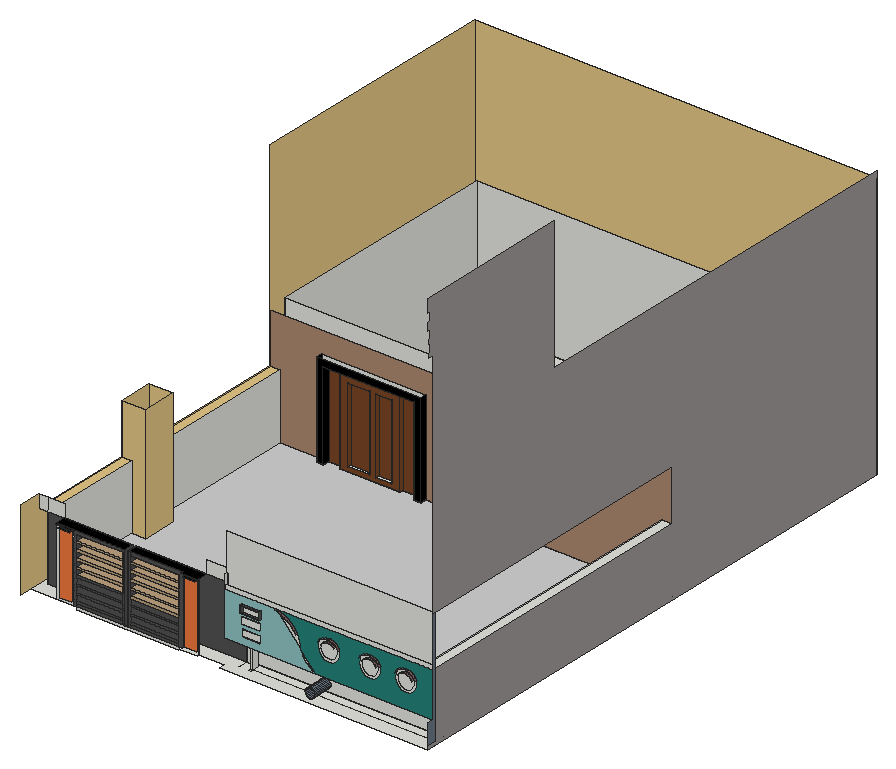
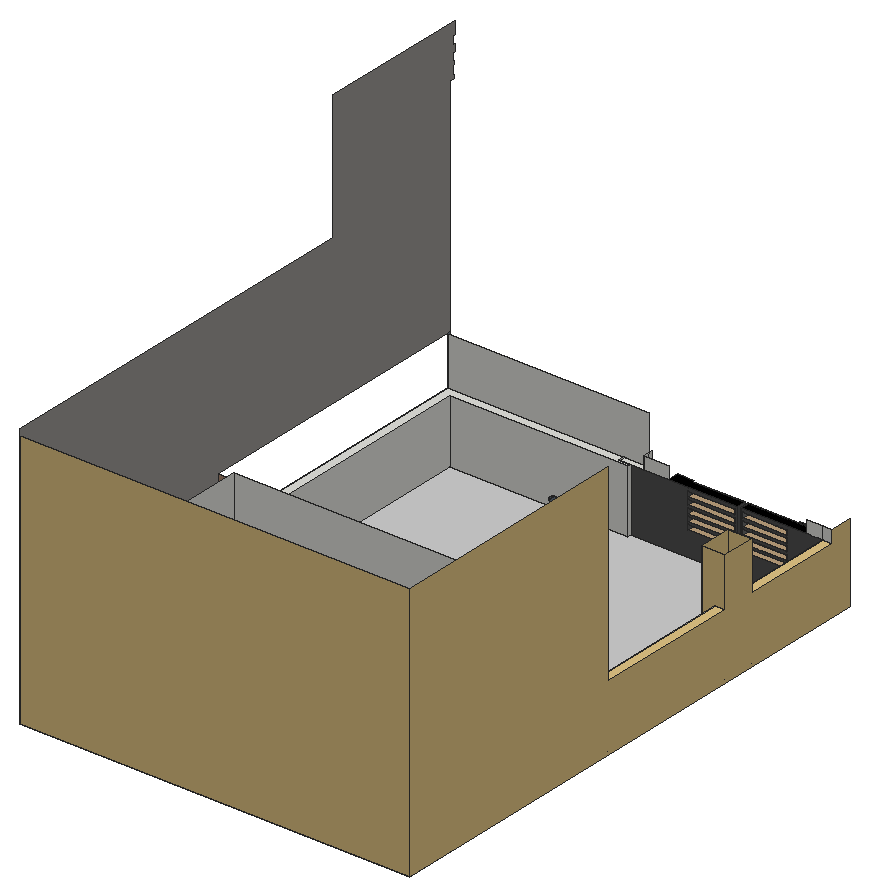
# SketchUp Ruby script. Lengths in inches.
U = 1.inch
M = Sketchup.active_model
def pt(a) = Geom::Point3d.new(a.map { |v| v * U })
def face(e, loops, mat)
  f = e.add_face(loops[0].map { |a| pt(a) })
  loops[1..].each { |l| e.add_face(l.map { |a| pt(a) }).erase! }
  f.material = f.back_material = mat if mat
  f
end
# faces: each face lists its corners as indices into pts; further lists are holes
def faces(e, pts, list, mat = nil) = list.each { |f| face(e, (f[0].is_a?(Array) ? f : [f]).map { |l| l.map { |i| pts[i] } }, mat) }
# xy, xz, yz: faces in a plane at the given z, y or x. An outline is a flat list of corners, or four numbers for a rectangle; further outlines are holes
def ring(l) = l.size == 4 ? [[l[0], l[1]], [l[2], l[1]], [l[2], l[3]], [l[0], l[3]]] : l.each_slice(2).to_a
def flat(e, list, mat, &to3) = list.each { |f| face(e, (f[0].is_a?(Array) ? f : [f]).map { |l| ring(l).map { |u, v| to3.(u, v) } }, mat) }
def xy(e, z, list, mat = nil) = flat(e, list, mat) { |x, y| [x, y, z] }
def xz(e, y, list, mat = nil) = flat(e, list, mat) { |x, z| [x, y, z] }
def yz(e, x, list, mat = nil) = flat(e, list, mat) { |y, z| [x, y, z] }
def lines(e, pts, list) = list.each { |a, b| e.add_line(pt(pts[a]), pt(pts[b])) }
# prism: a flat outline (further loops are holes) pulled along v
def prism(e, loops, v, mat = nil)
  f = face(e, loops, mat); d = Geom::Vector3d.new(v.map { |x| x * U })
  f.pushpull(f.normal.samedirection?(d) ? d.length : -d.length)
end
def box(e, o, s, mat = nil) = prism(e, [[o, [o[0] + s[0], o[1], o[2]], [o[0] + s[0], o[1] + s[1], o[2]], [o[0], o[1] + s[1], o[2]]]], [0, 0, s[2]], mat)
def at(x, y, z, deg = 0) = Geom::Transformation.translation(pt([x, y, z])) * Geom::Transformation.rotation(ORIGIN, Z_AXIS, deg.degrees)
def axes(o, x, y, z) = Geom::Transformation.new([*x, 0, *y, 0, *z, 0, *pt(o).to_a, 1])
def part(name) = M.definitions.add(name)
# library, detail: a bought-in or finely detailed component or shape, given as its bounding box
def library(name, o, s) = part(name).tap { |d| box(d.entities, o, s) }
def detail(e, o, s) = box(e.add_group.entities, o, s)
def put(e, d, t, mat = nil) = e.add_instance(d, t).tap { |i| i.material = mat if mat }
def group(e, t, mat = nil) = e.add_group.tap { |g| g.transformation = t; g.material = mat if mat }.entities
root = M.entities
M.materials.add("[0035_Tan]").color = [186, 159, 124]
M.materials.add("[0035_Tan]1").color = [210, 180, 140]
M.materials.add("[0085_Turquoise]").color = [37, 130, 120]
M.materials.add("[0089_PaleTurquoise]").color = [142, 193, 193]
M.materials.add("[0111_SlateGray]").color = [103, 117, 132]
M.materials.add("[0119_RosyBrown]1").color = [124, 95, 95]
M.materials.add("[0134_DimGray]").color = [105, 105, 105]
M.materials.add("[0135_DarkGray]").color = [81, 81, 81]
M.materials.add("[0137_Black]").color = [0, 0, 0]
M.materials.add("[Carrera Marble]").color = [207, 207, 207]
M.materials.add("[Cast-in-place Concrete]").color = [239, 119, 61]
M.materials.add("[Concrete Aggregate Smoke]").color = [154, 150, 148]
M.materials.add("[Stone Brushed Khaki]").color = [226, 197, 133]
M.materials.add("[Tile Veriegated Stone]").color = [171, 137, 112]
M.materials.add("[Wood Veneer 01]").color = [120, 70, 37]
xy(root,0,[[186.0625,645.11,186.0625,651.11,162.54,651.11,162.54,649.11,146.95,649.11,146.95,651.11,96.94,651.11,96.94,660.11,93.94,660.11,93.94,651.11,7,651.11,7,927.36,54.84,927.36,54.84,921.36,60.84,921.36,60.84,927.36,73.93,927.36,73.93,924.36,129.08,924.36,129.08,927.36,144.84,927.36,144.84,921.36,150.84,921.36,150.84,927.36,377.9375,927.36,377.9375,645.11],[93.94,651.11,96.94,660.11],[54.84,921.36,60.84,927.36],[144.84,921.36,150.84,927.36],[73.93,924.36,129.08,927.36],
  [[7,927.36,377.9375,1163.11],[16,933.36,358,1154.11]],[16,933.36,358,1154.11]])
xy(root,3,[[16,660.11,198.9375,660.11,198.9375,663.11,368.9375,663.11,368.9375,927.36,150.84,927.36,150.84,921.36,144.84,921.36,144.84,927.36,129.08,927.36,129.08,924.36,73.93,924.36,73.93,927.36,60.84,927.36,60.84,921.36,54.84,921.36,54.84,927.36,16,927.36,16,787.78,29,787.78,29,756.09,16,756.09]],"[Carrera Marble]")
xy(root,7.2,[[81.13,924.36,101.5,927.36],[107.04,924.36,121.875,927.36]])
xy(root,26.4,[[49.92,651.11,91.67,660.11],[99.37,651.11,143.95,660.11]],"[0035_Tan]")
xy(root,31.5,[[49.92,651.11,91.67,660.11]],"[0035_Tan]")
xy(root,31.5,[[99.37,651.11,143.95,660.11]],"[0035_Tan]1")
xy(root,33.52,[[49.92,651.11,91.67,660.11],[99.37,651.11,143.95,660.11]],"[0035_Tan]")
xy(root,38.625,[[49.92,651.11,91.67,660.11]],"[0035_Tan]")
xy(root,38.625,[[99.37,651.11,143.95,660.11]],"[0035_Tan]1")
xy(root,40.65,[[49.92,651.11,91.67,660.11],[99.37,651.11,143.95,660.11]],"[0035_Tan]")
xy(root,45.75,[[49.92,651.11,91.67,660.11]],"[0035_Tan]")
xy(root,45.75,[[99.37,651.11,143.95,660.11]],"[0035_Tan]1")
xy(root,47.77,[[49.92,651.11,91.67,660.11],[99.37,651.11,143.95,660.11]],"[0035_Tan]")
xy(root,49.0625,[[201.56,649.11,219.5,651.11]],"[0135_DarkGray]")
xy(root,49.82,[[202.32,649.11,218.74,651.11]],"[0135_DarkGray]")
xy(root,52.875,[[49.92,651.11,91.67,660.11],[99.37,651.11,143.95,660.11]],"[0035_Tan]")
xy(root,54.9,[[49.92,651.11,91.67,660.11],[99.37,651.11,143.95,660.11]],"[0035_Tan]")
xy(root,55.55,[[202.32,649.11,218.74,651.11]],"[0135_DarkGray]")
xy(root,56.3125,[[201.56,649.11,219.5,651.11]],"[0135_DarkGray]")
xy(root,60,[[49.92,651.11,91.67,660.11],[99.37,651.11,143.95,660.11]],"[0135_DarkGray]")
xy(root,60.7,[[33.63,649.11,44.62,651.11]],"[0137_Black]")
xy(root,60.93,[[149.02,649.11,160.48,651.11]],"[0137_Black]")
xy(root,63,[[186.0625,651.11,186.19,654.11],[186.19,651.11,209.625,654.11],[186.19,654.11,209.625,660.11],[209.625,654.11,377.9375,654.11,377.9375,927.36,368.9375,927.36,368.9375,663.11,198.9375,663.11,198.9375,660.11,209.625,660.11]])
xy(root,63,[[31.33,649.11,46.92,651.11],[146.95,649.11,162.54,649.11,162.54,651.11,162.58,651.11,162.58,660.11,96.94,660.11,96.94,651.11,146.95,651.11],[31.33,651.11,93.94,660.11]],"[0137_Black]")
xy(root,63,[[7,660.11,16,756.09],[7,787.78,16,927.36]],"[Stone Brushed Khaki]")
xz(root,651.11,[[49.92,-2.1,143.95,0],[[31.33,0,46.92,63],[33.63,2.3,44.62,60.7]],[162.54,0,162.58,63],[202.42,29.54,218.64,35.08],[282.78,38.68,284.61,39.03,286.28,39.84,287.68,41.0625,288.72,42.6,289.33,44.36,289.46,46.22,289.11,48.04,288.29,49.72,287.07,51.12,285.53,52.16,283.77,52.77,281.92,52.9,280.09,52.55,278.42,51.73,277.02,50.51,275.98,48.97,275.37,47.21,275.24,45.36,275.59,43.53,276.41,41.86,277.625,40.46,279.17,39.41,280.92,38.81],
  [320.72,38.68,322.54,39.03,324.22,39.84,325.62,41.0625,326.66,42.6,327.27,44.36,327.4,46.22,327.05,48.04,326.23,49.72,325.01,51.12,323.47,52.16,321.71,52.77,319.86,52.9,318.03,52.55,316.36,51.73,314.95,50.51,313.91,48.97,313.31,47.21,313.18,45.36,313.53,43.53,314.34,41.86,315.5625,40.46,317.1,39.41,318.86,38.81],[353.97,38.68,355.79,39.03,357.47,39.84,358.87,41.0625,359.91,42.6,360.52,44.36,360.65,46.22,360.3,48.04,359.48,49.72,358.26,51.12,356.72,52.16,354.96,52.77,353.11,52.9,351.28,52.55,349.61,51.73,348.2,50.51,347.16,48.97,346.56,47.21,346.43,45.36,346.78,43.53,347.59,41.86,348.8125,40.46,350.35,39.41,352.11,38.81],[202.31,39.62,218.75,45.375],[202.32,49.82,218.74,55.55],[186.0625,63,377.9375,67.2]])
xz(root,651.11,[[99.37,24.375,143.95,26.4],[49.92,31.5,91.67,33.52],[99.37,31.5,143.95,33.52],[49.92,38.625,91.67,40.65],[99.37,38.625,143.95,40.65],
  [49.92,45.75,91.67,47.77],[99.37,45.75,143.95,47.77],[49.92,52.875,91.67,54.9],[99.37,52.875,143.95,54.9]],"[0035_Tan]")
xz(root,651.11,[[[270.01,22.19,377.9375,22.19,377.9375,63,233.66,63,236.68,62.29,239.6,61.26,242.39,59.9,245.01,58.24,247.43,56.31,249.62,54.11,251.55,51.68,253.19,49.06,254.54,46.26,255.56,43.34,256.26,40.32,256.61,37.24,256.72,37.33,270.11,22.28],[282.96,35.68,280.32,35.87,277.83,36.73,275.64,38.21,273.9,40.21,272.75,42.58,272.24,45.18,272.43,47.8125,273.29,50.3125,274.77,52.5,276.77,54.24,279.14,55.39,281.74,55.9,284.375,55.71,286.875,54.85,289.0625,53.37,290.8,51.37,291.95,48.99,292.46,46.4,292.27,43.76,291.41,41.26,289.93,39.07,287.93,37.34,285.56,36.18],[320.9,35.68,318.26,35.87,315.76,36.73,313.57,38.21,311.84,40.21,310.68,42.58,310.18,45.18,310.37,47.8125,311.23,50.3125,312.71,52.5,314.7,54.24,317.08,55.39,319.68,55.9,322.3125,55.71,324.8125,54.85,327,53.37,328.73,51.37,329.89,48.99,330.39,46.4,330.21,43.76,329.35,41.26,327.87,39.07,325.87,37.34,323.49,36.18],[354.15,35.68,351.51,35.87,349.01,36.73,346.82,38.21,345.09,40.21,343.93,42.58,343.43,45.18,343.62,47.8125,344.48,50.3125,345.96,52.5,347.95,54.24,350.33,55.39,352.93,55.9,355.5625,55.71,358.0625,54.85,360.25,53.37,361.98,51.37,363.14,48.99,363.64,46.4,363.46,43.76,362.6,41.26,361.12,39.07,359.12,37.34,356.74,36.18]]],"[0085_Turquoise]")
xz(root,651.11,[[[186.0625,22.19,270.01,22.19,268.33,22.75,266.71,23.47,265.17,24.34,263.71,25.35,262.36,26.49,261.12,27.76,260,29.14,259.02,30.61,258.1875,32.18,257.5,33.8125,256.97,35.5,256.61,37.24,233.66,63,186.0625,63],[201.56,49.0625,219.5,56.3125],[201.56,38.875,219.5,46.125],[201.56,28.6875,219.5,35.9375]]],"[0089_PaleTurquoise]")
xz(root,651.11,[[46.92,0,49.92,0,49.92,60,91.67,60,91.67,0,93.94,0,93.94,63,46.92,63],[49.92,0,91.67,3],[96.94,0,99.37,63],[143.95,0,146.95,0,146.95,63,99.37,63,99.37,60,143.95,60],[99.37,0,143.95,3],
  [49.92,3,91.67,5.02],[99.37,3,143.95,5.02],[49.92,5.02,91.67,10.125],[99.37,5.02,143.95,10.125],[49.92,10.125,91.67,12.15],
  [99.37,10.125,143.95,12.15],[49.92,12.15,91.67,17.25],[99.37,12.15,143.95,17.25],[49.92,17.25,91.67,19.27],[99.37,17.25,143.95,19.27],
  [49.92,19.27,91.67,24.375],[99.37,19.27,143.95,24.375],[49.92,24.375,91.67,26.4]],"[0135_DarkGray]")
xz(root,651.11,[[149.02,2.07,160.48,60.93],[33.63,2.3,44.62,60.7]],"[Cast-in-place Concrete]")
xz(root,654.11,[[207.9375,3,209.625,63],[186.0625,63,186.19,75],[186.19,63,186.19,75,186.0625,75,186.0625,109.5,377.9375,109.5,377.9375,63]])
xz(root,660.11,[[93.94,0,96.94,3],[198.9375,3,209.625,63],[7,63,16,75],[16,63,31.33,75],[162.58,63,186.19,75]])
xz(root,660.11,[[[16,3,93.94,63],[49.92,54.9,91.67,60],[49.92,47.77,91.67,52.875],[49.92,40.65,91.67,45.75],[49.92,33.52,91.67,38.625],[49.92,26.4,91.67,31.5]],[[96.94,3,198.9375,63],[99.37,26.4,143.95,31.5],[99.37,54.9,143.95,60],[99.37,47.77,143.95,52.875],[99.37,40.65,143.95,45.75],[99.37,33.52,143.95,38.625]]],"[0135_DarkGray]")
xz(root,663.11,[[[198.9375,3,368.9375,63],[269.68,4.18,270.85,4.33,271.93,4.78,272.87,5.5,273.58,6.43,274.03,7.52,274.18,8.68,274.03,9.85,273.58,10.93,272.87,11.86,271.93,12.58,270.85,13.03,269.68,13.18,268.52,13.03,267.43,12.58,266.5,11.86,265.79,10.93,265.34,9.85,265.18,8.68,265.34,7.52,265.79,6.43,266.5,5.5,267.43,4.78,268.52,4.33]]])
xz(root,756.09,[[16,3,29,3,29,109.5,7,109.5,7,63,16,63]],"[Stone Brushed Khaki]")
xz(root,787.78,[[16,3,16,63,7,63,7,109.5,29,109.5,29,3]],"[Stone Brushed Khaki]")
xz(root,921.36,[[54.84,0,60.84,3],[144.84,0,150.84,3]])
xz(root,921.36,[[54.84,3,60.84,3,60.84,84,144.84,84,144.84,3,150.84,3,150.84,90,54.84,90]],"[0137_Black]")
xz(root,924.36,[[73.93,0,129.08,3]])
xz(root,924.36,[[[73.93,3,129.08,84],[81.13,7.2,101.5,76.8],[107.04,7.2,121.875,76.8]]],"[Wood Veneer 01]")
xz(root,927.36,[[60.84,0,73.93,3],[129.08,0,144.84,3],[150.84,0,367,3]])
xz(root,927.36,[[16,3,54.84,3,54.84,90,150.84,90,150.84,3,368.9375,3,368.9375,63,377.9375,63,377.9375,109.5,7,109.5,7,63,16,63]],"[Tile Veriegated Stone]")
xz(root,927.36,[[60.84,3,73.93,84],[129.08,3,144.84,84],[81.13,7.2,101.5,76.8],[107.04,7.2,121.875,76.8]],"[Wood Veneer 01]")
xz(root,933.36,[[16,0,358,120]])
xz(root,1154.11,[[16,0,358,120]])
xz(root,1163.11,[[7,0,377.9375,245.51]],"[Stone Brushed Khaki]")
yz(root,7,[[639.11,0,639.11,75,660.11,75,660.11,63,756.09,63,756.09,109.5,787.78,109.5,787.78,63,927.36,63,927.36,245.51,1163.11,245.51,1163.11,0]],"[Stone Brushed Khaki]")
yz(root,16,[[933.36,0,1154.11,120],[660.11,3,756.09,63],[787.78,3,927.36,63]])
yz(root,29,[[756.09,3,787.78,109.5]],"[Stone Brushed Khaki]")
yz(root,49.92,[[651.11,26.4,660.11,31.5],[651.11,33.52,660.11,38.625],[651.11,40.65,660.11,45.75],[651.11,47.77,660.11,52.875],[651.11,54.9,660.11,60]],"[0135_DarkGray]")
yz(root,54.84,[[921.36,0,927.36,3]])
yz(root,54.84,[[921.36,3,927.36,90]],"[0137_Black]")
yz(root,60.84,[[921.36,0,927.36,3]])
yz(root,60.84,[[921.36,3,927.36,84]],"[0137_Black]")
yz(root,73.93,[[924.36,0,927.36,3]])
yz(root,73.93,[[924.36,3,927.36,84]],"[Wood Veneer 01]")
yz(root,81.13,[[924.36,7.2,927.36,76.8]],"[Wood Veneer 01]")
yz(root,91.67,[[651.11,26.4,660.11,31.5],[651.11,33.52,660.11,38.625],[651.11,40.65,660.11,45.75],[651.11,47.77,660.11,52.875],[651.11,54.9,660.11,60]],"[0134_DimGray]")
yz(root,93.94,[[651.11,0,660.11,63]],"[0135_DarkGray]")
yz(root,96.94,[[651.11,0,660.11,63]],"[0135_DarkGray]")
yz(root,99.37,[[651.11,26.4,660.11,31.5],[651.11,33.52,660.11,38.625],[651.11,40.65,660.11,45.75],[651.11,47.77,660.11,52.875],[651.11,54.9,660.11,60]],"[0135_DarkGray]")
yz(root,101.5,[[924.36,7.2,927.36,76.8]],"[Wood Veneer 01]")
yz(root,107.04,[[924.36,7.2,927.36,76.8]],"[Wood Veneer 01]")
yz(root,121.875,[[924.36,7.2,927.36,76.8]],"[Wood Veneer 01]")
yz(root,129.08,[[924.36,0,927.36,3]])
yz(root,129.08,[[924.36,3,927.36,84]],"[Wood Veneer 01]")
yz(root,143.95,[[651.11,26.4,660.11,31.5],[651.11,33.52,660.11,38.625],[651.11,40.65,660.11,45.75],[651.11,47.77,660.11,52.875],[651.11,54.9,660.11,60]],"[0135_DarkGray]")
yz(root,144.84,[[921.36,0,927.36,3]])
yz(root,144.84,[[921.36,3,927.36,84]],"[0137_Black]")
yz(root,150.84,[[921.36,0,927.36,3]])
yz(root,150.84,[[921.36,3,927.36,90]],"[0137_Black]")
yz(root,186.0625,[[651.11,63,654.11,75]])
yz(root,186.19,[[654.11,63,660.11,75]])
yz(root,198.9375,[[660.11,3,663.11,63]])
yz(root,201.56,[[649.11,49.0625,651.11,56.3125]])
yz(root,202.32,[[649.11,49.82,651.11,55.55]],"[0135_DarkGray]")
yz(root,209.625,[[654.11,3,660.11,63]])
yz(root,218.74,[[649.11,49.82,651.11,55.55]],"[0135_DarkGray]")
yz(root,219.5,[[649.11,49.0625,651.11,56.3125]],"[0135_DarkGray]")
yz(root,358,[[933.36,0,1154.11,120]])
yz(root,368.9375,[[663.11,3,927.36,63]])
yz(root,377.9375,[[645.11,3,654.11,3,654.11,109.5,651.11,109.5,651.11,22.19,645.11,22.19]],"[0111_SlateGray]")
yz(root,377.9375,[[645.11,0,1163.11,0,1163.11,251.36,791.05,251.36,791.05,372.74,645.43,372.74,645.43,360.74,648.43,360.74,648.43,352.6875,645.43,352.6875,645.43,346.17,648.43,346.17,648.43,338.52,646.43,338.52,646.43,335.1875,648.43,335.1875,648.43,326.96,646.43,326.96,646.43,323.31,651.11,323.31,651.11,109.5,927.36,109.5,927.36,63,654.11,63,654.11,3,645.11,3]],"[Concrete Aggregate Smoke]")
p = [[268.52,645.11,4.33],[269.68,645.11,4.18],[269.68,663.11,4.18],[268.52,663.11,4.33],[270.85,645.11,4.33],[270.85,663.11,4.33],
  [267.43,645.11,4.78],[267.43,663.11,4.78],[271.93,645.11,4.78],[271.93,663.11,4.78],[266.5,645.11,5.5],[266.5,663.11,5.5],
  [272.87,645.11,5.5],[272.87,663.11,5.5],[265.79,645.11,6.43],[265.79,663.11,6.43],[273.58,645.11,6.43],[273.58,663.11,6.43],
  [265.34,645.11,7.52],[265.34,663.11,7.52],[274.03,645.11,7.52],[274.03,663.11,7.52],[265.18,645.11,8.68],[265.18,663.11,8.68],
  [274.18,645.11,8.68],[274.18,663.11,8.68],[265.34,645.11,9.85],[265.34,663.11,9.85],[274.03,645.11,9.85],[274.03,663.11,9.85],
  [265.79,645.11,10.93],[265.79,663.11,10.93],[273.58,645.11,10.93],[273.58,663.11,10.93],[266.5,645.11,11.86],[266.5,663.11,11.86],
  [272.87,645.11,11.86],[272.87,663.11,11.86],[267.43,645.11,12.58],[267.43,663.11,12.58],[271.93,645.11,12.58],[271.93,663.11,12.58],
  [268.52,645.11,13.03],[268.52,663.11,13.03],[270.85,645.11,13.03],[270.85,663.11,13.03],[269.68,645.11,13.18],[269.68,663.11,13.18],
  [326.23,651.11,49.72],[327.05,651.11,48.04],[327.05,649.11,48.04],[326.23,649.11,49.72],[359.48,651.11,49.72],[360.3,651.11,48.04],
  [360.3,649.11,48.04],[359.48,649.11,49.72],[275.98,651.11,48.97],[277.02,651.11,50.51],[277.02,649.11,50.51],[275.98,649.11,48.97],
  [291.95,651.11,48.99],[290.8,651.11,51.37],[290.8,649.11,51.37],[291.95,649.11,48.99],[313.91,651.11,48.97],[314.95,651.11,50.51],
  [314.95,649.11,50.51],[313.91,649.11,48.97],[329.89,651.11,48.99],[328.73,651.11,51.37],[328.73,649.11,51.37],[329.89,649.11,48.99],
  [347.16,651.11,48.97],[348.2,651.11,50.51],[348.2,649.11,50.51],[347.16,649.11,48.97],[363.14,651.11,48.99],[361.98,651.11,51.37],
  [361.98,649.11,51.37],[363.14,649.11,48.99],[253.19,651.11,49.06],[251.55,651.11,51.68],[251.55,649.11,51.68],[253.19,649.11,49.06],
  [287.07,651.11,51.12],[288.29,651.11,49.72],[288.29,649.11,49.72],[287.07,649.11,51.12],[325.01,651.11,51.12],[325.01,649.11,51.12],
  [358.26,651.11,51.12],[358.26,649.11,51.12],[274.77,651.11,52.5],[273.29,651.11,50.3125],[273.29,649.11,50.3125],[274.77,649.11,52.5],
  [312.71,651.11,52.5],[311.23,651.11,50.3125],[311.23,649.11,50.3125],[312.71,649.11,52.5],[345.96,651.11,52.5],[344.48,651.11,50.3125],
  [344.48,649.11,50.3125],[345.96,649.11,52.5],[278.42,651.11,51.73],[278.42,649.11,51.73],[316.36,651.11,51.73],[316.36,649.11,51.73],
  [349.61,651.11,51.73],[349.61,649.11,51.73],[285.53,651.11,52.16],[285.53,649.11,52.16],[323.47,651.11,52.16],[323.47,649.11,52.16],
  [356.72,651.11,52.16],[356.72,649.11,52.16],[289.0625,651.11,53.37],[289.0625,649.11,53.37],[327,651.11,53.37],[327,649.11,53.37],
  [360.25,651.11,53.37],[360.25,649.11,53.37],[249.62,651.11,54.11],[249.62,649.11,54.11],[280.09,651.11,52.55],[280.09,649.11,52.55],
  [318.03,651.11,52.55],[318.03,649.11,52.55],[351.28,651.11,52.55],[351.28,649.11,52.55],[283.77,651.11,52.77],[283.77,649.11,52.77],
  [321.71,651.11,52.77],[321.71,649.11,52.77],[354.96,651.11,52.77],[354.96,649.11,52.77],[276.77,651.11,54.24],[276.77,649.11,54.24],
  [281.92,651.11,52.9],[281.92,649.11,52.9],[314.7,651.11,54.24],[314.7,649.11,54.24],[319.86,651.11,52.9],[319.86,649.11,52.9],
  [347.95,651.11,54.24],[347.95,649.11,54.24],[353.11,651.11,52.9],[353.11,649.11,52.9],[286.875,651.11,54.85],[286.875,649.11,54.85],
  [324.8125,651.11,54.85],[324.8125,649.11,54.85],[358.0625,651.11,54.85],[358.0625,649.11,54.85],[247.43,651.11,56.31],[247.43,649.11,56.31],
  [279.14,651.11,55.39],[279.14,649.11,55.39],[317.08,651.11,55.39],[317.08,649.11,55.39],[350.33,651.11,55.39],[350.33,649.11,55.39],
  [284.375,651.11,55.71],[284.375,649.11,55.71],[322.3125,651.11,55.71],[322.3125,649.11,55.71],[355.5625,651.11,55.71],[355.5625,649.11,55.71],
  [281.74,651.11,55.9],[281.74,649.11,55.9],[319.68,651.11,55.9],[319.68,649.11,55.9],[352.93,651.11,55.9],[352.93,649.11,55.9],
  [245.01,651.11,58.24],[245.01,649.11,58.24],[242.39,651.11,59.9],[242.39,649.11,59.9],[239.6,651.11,61.26],[239.6,649.11,61.26],
  [236.68,651.11,62.29],[236.68,649.11,62.29],[233.66,651.11,63],[233.66,649.11,63],[7,927.36,3],[16,927.36,3],
  [16,787.78,3],[7,787.78,3],[16,927.59,3],[198.9375,660.11,3],[198.9375,651.11,3],[7,756.09,3],
  [16,756.09,3],[207.9375,654.11,3],[207.9375,651.11,3],[209.625,654.11,3],[209.625,651.11,3],[377.9375,927.36,3],
  [368.9375,927.36,3],[368.9375,663.11,3],[377.9375,663.11,3],[377.9375,654.11,3]]
faces(root,p,[[0,1,2,3],[1,4,5,2],[6,0,3,7],[4,8,9,5],[10,6,7,11],[8,12,13,9],[14,10,11,15],[12,16,17,13],
  [18,14,15,19],[16,20,21,17],[22,18,19,23],[20,24,25,21],[26,22,23,27],[24,28,29,25],[30,26,27,31],[28,32,33,29],
  [34,30,31,35],[32,36,37,33],[38,34,35,39],[36,40,41,37],[42,38,39,43],[40,44,45,41],[46,42,43,47],[44,46,47,45]],"[0111_SlateGray]")
faces(root,p,[[48,49,50,51],[52,53,54,55],[56,57,58,59],[60,61,62,63],[64,65,66,67],[68,69,70,71],[72,73,74,75],[76,77,78,79],
  [80,81,82,83],[84,85,86,87],[88,48,51,89],[90,52,55,91],[92,93,94,95],[96,97,98,99],[100,101,102,103],[57,104,105,58],
  [65,106,107,66],[73,108,109,74],[110,84,87,111],[112,88,89,113],[114,90,91,115],[61,116,117,62],[69,118,119,70],[77,120,121,78],
  [81,122,123,82],[104,124,125,105],[106,126,127,107],[108,128,129,109],[130,110,111,131],[132,112,113,133],[134,114,115,135],[136,92,95,137],
  [124,138,139,125],[140,96,99,141],[126,142,143,127],[144,100,103,145],[128,146,147,129],[138,130,131,139],[142,132,133,143],[146,134,135,147],
  [116,148,149,117],[118,150,151,119],[120,152,153,121],[122,154,155,123],[156,136,137,157],[158,140,141,159],[160,144,145,161],[148,162,163,149],
  [150,164,165,151],[152,166,167,153],[168,156,157,169],[170,158,159,171],[172,160,161,173],[162,168,169,163],[164,170,171,165],[166,172,173,167],
  [154,174,175,155],[174,176,177,175],[176,178,179,177],[178,180,181,179],[180,182,183,181]],"[0119_RosyBrown]1")
lines(root,p,[[184,185],[186,187],[188,185],[189,190],[191,192],[193,194],[195,196],[197,198],[199,200],[201,195]])
